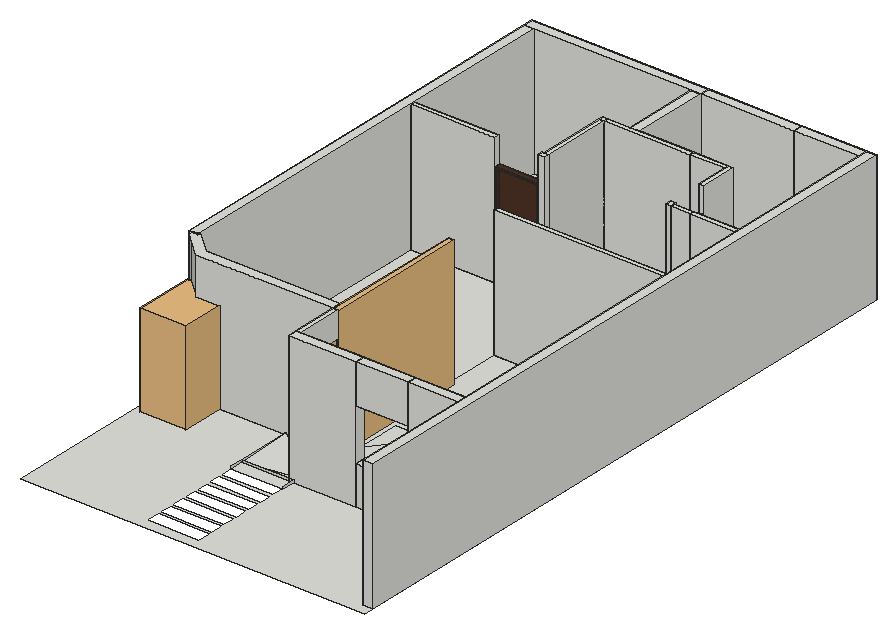
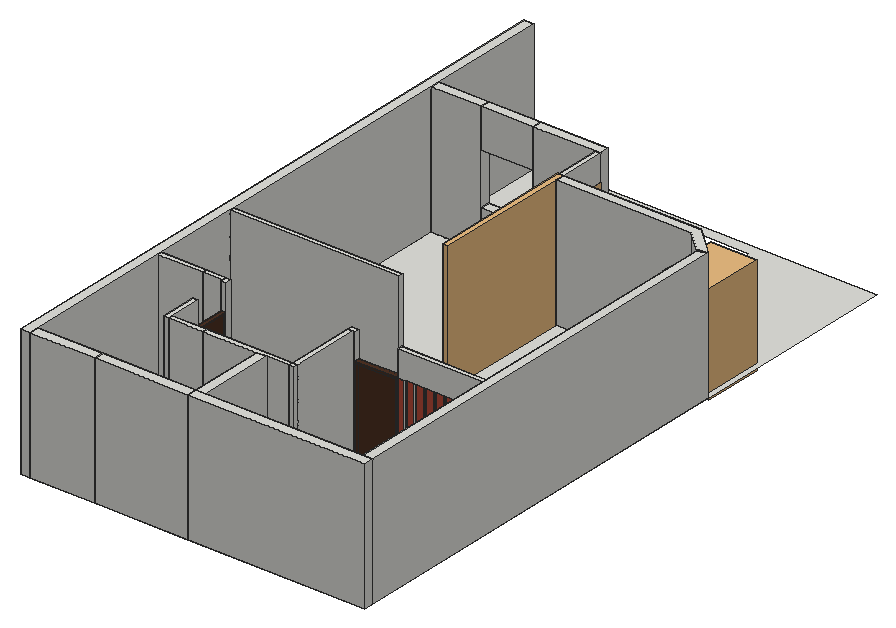
# SketchUp Ruby script. Lengths in inches.
U = 1.inch
M = Sketchup.active_model
def pt(a) = Geom::Point3d.new(a.map { |v| v * U })
def face(e, loops, mat)
  f = e.add_face(loops[0].map { |a| pt(a) })
  loops[1..].each { |l| e.add_face(l.map { |a| pt(a) }).erase! }
  f.material = f.back_material = mat if mat
  f
end
# faces: each face lists its corners as indices into pts; further lists are holes
def faces(e, pts, list, mat = nil) = list.each { |f| face(e, (f[0].is_a?(Array) ? f : [f]).map { |l| l.map { |i| pts[i] } }, mat) }
# xy, xz, yz: faces in a plane at the given z, y or x. An outline is a flat list of corners, or four numbers for a rectangle; further outlines are holes
def ring(l) = l.size == 4 ? [[l[0], l[1]], [l[2], l[1]], [l[2], l[3]], [l[0], l[3]]] : l.each_slice(2).to_a
def flat(e, list, mat, &to3) = list.each { |f| face(e, (f[0].is_a?(Array) ? f : [f]).map { |l| ring(l).map { |u, v| to3.(u, v) } }, mat) }
def xy(e, z, list, mat = nil) = flat(e, list, mat) { |x, y| [x, y, z] }
def xz(e, y, list, mat = nil) = flat(e, list, mat) { |x, z| [x, y, z] }
def yz(e, x, list, mat = nil) = flat(e, list, mat) { |y, z| [x, y, z] }
def lines(e, pts, list) = list.each { |a, b| e.add_line(pt(pts[a]), pt(pts[b])) }
# prism: a flat outline (further loops are holes) pulled along v
def prism(e, loops, v, mat = nil)
  f = face(e, loops, mat); d = Geom::Vector3d.new(v.map { |x| x * U })
  f.pushpull(f.normal.samedirection?(d) ? d.length : -d.length)
end
def box(e, o, s, mat = nil) = prism(e, [[o, [o[0] + s[0], o[1], o[2]], [o[0] + s[0], o[1] + s[1], o[2]], [o[0], o[1] + s[1], o[2]]]], [0, 0, s[2]], mat)
def at(x, y, z, deg = 0) = Geom::Transformation.translation(pt([x, y, z])) * Geom::Transformation.rotation(ORIGIN, Z_AXIS, deg.degrees)
def axes(o, x, y, z) = Geom::Transformation.new([*x, 0, *y, 0, *z, 0, *pt(o).to_a, 1])
def part(name) = M.definitions.add(name)
# library, detail: a bought-in or finely detailed component or shape, given as its bounding box
def library(name, o, s) = part(name).tap { |d| box(d.entities, o, s) }
def detail(e, o, s) = box(e.add_group.entities, o, s)
def put(e, d, t, mat = nil) = e.add_instance(d, t).tap { |i| i.material = mat if mat }
def group(e, t, mat = nil) = e.add_group.tap { |g| g.transformation = t; g.material = mat if mat }.entities
root = M.entities
M.materials.add("Marc_Wrist").color = [188, 79, 61]
M.materials.add("Material1").color = [58, 110, 58]
M.materials.add("Material10").color = [48, 100, 38]
M.materials.add("Material3").color = [68, 110, 58]
M.materials.add("Material4").color = [48, 90, 38]
M.materials.add("Material5").color = [68, 110, 48]
M.materials.add("Material6").color = [48, 90, 48]
M.materials.add("Material8").color = [58, 90, 38]
M.materials.add("Material9").color = [68, 100, 58]
M.materials.add("Polis06_194").color = [79, 50, 36]
M.materials.add("ThomThom - ShoesRubber2").color = [10, 10, 10]
M.materials.add("[Color_E04]").color = [255, 255, 153]
M.materials.add("[Wood Cherry Original]").color = [152, 86, 42]
c1 = part("grass00")
p = [[-0.6875,0.15,0],[-0.56,0.08,5.52],[-0.04,0.03,2.76],[0.48,-0.02,0],[0.35,-0.02,5.52],[-0.1,-0.14,5.52],
  [-0.12,0.65,8.37],[-0.42,0.65,8.37]]
faces(c1.entities,p,[[0,1,2,3],[3,2,4],[1,5,2],[5,4,2],[1,6,5],[4,5,6],[7,6,1]])
c2 = part("Group16\#1")
put(c2.entities,c1,axes([1.44,-0.61,-0.01],[0.05352,0.12609,0],[-0.10704,0.04543,0.07239],[0.06664,-0.02828,0.11628]),"Material6")
put(c2.entities,c1,axes([0.76,-0.15,-0.01],[0.04676,0.24062,0],[-0.23162,0.04501,0.06642],[0.0652,-0.01267,0.23595]),"Material3")
put(c2.entities,c1,axes([0.79,0.01,-0.01],[-0.00606,0.34651,0],[-0.34381,-0.00602,0.0432],[0.04319,0.00076,0.34386]))
put(c2.entities,c1,axes([1,0.23,-0.01],[-0.07192,0.31144,0],[-0.28722,-0.06632,0.1236],[0.12043,0.02781,0.29478]),"Material5")
put(c2.entities,c1,axes([1.66,0.77,-0.01],[-0.13828,0.29651,0],[-0.21551,-0.1005,0.22471],[0.20365,0.09498,0.23779]),"Material10")
put(c2.entities,c1,axes([0.6875,0.52,-0.01],[-0.18126,0.24051,0],[-0.22746,-0.17142,0.09788],[0.07817,0.05891,0.28481]),"Material5")
put(c2.entities,c1,axes([0.68,0.78,-0.01],[-0.215,0.18688,0],[-0.12385,-0.14248,0.21334],[0.13995,0.16101,0.18878]),"Material3")
put(c2.entities,c1,axes([0.56,1,-0.01],[-0.13756,0.07624,0],[-0.06159,-0.11112,0.0927],[0.04494,0.08108,0.12705]),"Material5")
put(c2.entities,c1,axes([0.2,0.64,-0.01],[-0.23729,0.07254,0],[-0.05711,-0.18681,0.153],[0.04473,0.14632,0.19535]),"Material10")
put(c2.entities,c1,axes([0.0625,0.72,-0.01],[-0.28874,0.02525,0],[-0.02179,-0.24916,0.14647],[0.01276,0.14591,0.25012]),"Material3")
put(c2.entities,c1,axes([-0.08,0.62,-0.01],[-0.34089,-0.04187,0],[0.03255,-0.26504,0.216],[-0.02633,0.21439,0.26703]),"Material10")
put(c2.entities,c1,axes([-0.34,0.98,-0.01],[-0.14314,-0.0493,0],[0.04397,-0.12769,0.06843],[-0.02228,0.0647,0.13505]),"Material10")
put(c2.entities,c1,axes([-0.87,1.45,-0.01],[-0.23488,-0.14114,0],[0.13761,-0.22901,0.06087],[-0.03135,0.05217,0.26717]))
put(c2.entities,c1,axes([-0.72,0.77,-0.01],[-0.14208,-0.13251,0],[0.07209,-0.0773,0.16301],[-0.11118,0.11922,0.1057]),"Material10")
put(c2.entities,c1,axes([-0.62,0.43,-0.01],[-0.14845,-0.21203,0],[0.18654,-0.13061,0.12304],[-0.10079,0.07057,0.22772]),"Material3")
put(c2.entities,c1,axes([-0.68,0.29,-0.01],[-0.13639,-0.32136,0],[0.31723,-0.13464,0.05579],[-0.05136,0.0218,0.34462]),"Material4")
put(c2.entities,c1,axes([-0.64,0.125,-0.01],[-0.0458,-0.23569,0],[0.22124,-0.043,0.08276],[-0.08124,0.01579,0.22538]),"Material1")
put(c2.entities,c1,axes([-1.6,-0.03,-0.01],[0.00576,-0.32897,0],[0.27526,0.00482,0.18018],[-0.18015,-0.00315,0.2753]),"Material5")
put(c2.entities,c1,axes([-1.36,-0.31,-0.01],[0.05718,-0.24765,0],[0.18172,0.04196,0.17267],[-0.16825,-0.03885,0.1865]),"Material10")
put(c2.entities,c1,axes([-1.54,-0.72,-0.01],[0.06537,-0.14017,0],[0.13555,0.06321,0.03939],[-0.0357,-0.01665,0.14956]))
put(c2.entities,c1,axes([-1.19,-0.9,-0.01],[0.09597,-0.12735,0],[0.11214,0.08451,0.07557],[-0.06035,-0.04548,0.14042]),"Material9")
put(c2.entities,c1,axes([-0.47,-0.54,-0.01],[0.11588,-0.10072,0],[0.0618,0.0711,0.12124],[-0.07953,-0.0915,0.0942]))
put(c2.entities,c1,axes([-0.47,-0.84,-0.01],[0.11927,-0.0661,0],[0.06603,0.11913,0.00646],[-0.00313,-0.00565,0.13621]),"Material5")
put(c2.entities,c1,axes([-0.38,-1.24,-0.01],[0.28037,-0.08571,0],[0.0618,0.20215,0.20315],[-0.05939,-0.19428,0.21139]),"Material9")
put(c2.entities,c1,axes([-0.06,-0.66,-0.01],[0.22719,-0.01987,0],[0.01247,0.14255,0.17758],[-0.01547,-0.17691,0.1431]),"Material8")
put(c2.entities,c1,axes([0.11,-0.89,-0.01],[0.14882,0.01828,0],[-0.01058,0.08611,0.12229],[0.01491,-0.12138,0.08676]),"Material6")
put(c2.entities,c1,axes([0.25,-0.72,-0.01],[0.20481,0.07053,0],[-0.06206,0.18022,0.10291],[0.03351,-0.0973,0.1906]),"Material6")
put(c2.entities,c1,axes([0.85,-1.42,-0.01],[0.16481,0.09904,0],[-0.09472,0.15762,0.05616],[0.02893,-0.04814,0.18389]),"Material5")
put(c2.entities,c1,axes([1.01,-1.09,-0.01],[0.21858,0.20385,0],[-0.17495,0.1876,0.15339],[0.10462,-0.11218,0.25652]),"Material10")
put(c2.entities,c1,axes([1.01,-0.71,-0.01],[0.08733,0.12473,0],[-0.06445,0.04512,0.13037],[0.1068,-0.07477,0.07867]),"Material6")
c3 = part("Group15\#1")
put(c3.entities,c2,at(0,0,0))
c4 = part("3darcstudiotree_grass00\#1")
put(c4.entities,c3,at(0,0,0))
c5 = library("DD LT 2",[0,0,0],[47.24,4.7,78.74])
c6 = library("Group\#96",[-3.28,-8.3,0],[42.48,54.86,91.86])
c7 = library("Group\#9",[0,0,0],[5.16,133,120])
c8 = part("Group\#23")
box(c8.entities,[0,0,0],[12.05,39.48,6])
c9 = part("Flush door")
xy(c9.entities,0,[[0,0,4.72,1.18],[0,34.25,4.72,35.43]],"Polis06_194")
xy(c9.entities,85.26,[[0,1.18,4.72,34.25]],"Polis06_194")
xy(c9.entities,86.61,[[0,0,4.72,35.43]],"Polis06_194")
xz(c9.entities,0,[[0,0,4.72,86.61]],"Polis06_194")
xz(c9.entities,1.18,[[0,0,2.36,85.26],[2.36,0,4.72,85.26]],"Polis06_194")
xz(c9.entities,34.25,[[0,0,4.72,85.26]],"Polis06_194")
xz(c9.entities,35.43,[[0,0,4.72,86.61]],"Polis06_194")
yz(c9.entities,0,[[0,0,1.18,86.61],[34.25,0,35.43,86.61],[1.18,85.26,34.25,86.61]],"Polis06_194")
yz(c9.entities,2.36,[[1.18,0,34.25,0,34.25,85.21,1.18,85.26]],"Polis06_194")
yz(c9.entities,4.72,[[0,0,1.18,86.61],[34.25,0,35.43,86.61],[1.18,85.26,34.25,86.61]],"Polis06_194")
xy(root,0,[[[28.97,48,346.97,638.5],[138.47,142.5,138.47,166.5,191.85,175.5,181.97,175.5,181.97,403.5,337.97,403.5,337.97,175.5,223.49,175.5,181.66,166.5,186.47,166.5,186.47,142.5],[138.47,57,186.47,70.5],[138.47,72.5,186.47,84.5],[138.47,86.5,186.47,98.5],[138.47,100.5,186.47,112.5],[138.47,114.5,186.47,126.5],[138.47,128.5,186.47,140.5]],[138.47,154.5,186.47,166.5],[138.47,166.5,191.85,175.5,223.49,175.5,181.66,166.5],[181.97,175.5,181.97,403.5,337.97,403.5,337.97,175.5,223.49,175.5,223.49,277.625,191.85,277.625,191.85,175.5],[191.85,175.5,223.49,277.625]])
xz(root,166.5,[[138.47,0,181.66,2],[181.66,0,186.47,2]])
yz(root,138.47,[[154.5,0,166.5,2],[166.5,0,166.5,2,218,2]])
yz(root,186.47,[[154.5,0,166.5,2]])
p = [[191.85,175.5,0],[138.47,166.5,0],[138.47,218,2],[181.66,166.5,0],[223.49,175.5,0],[181.66,166.5,2],
  [223.49,277.625,0],[181.66,218,2]]
faces(root,p,[[0,1,2],[3,4,5],[5,4,6,7]])
put(root,c4,axes([269.28,156.1,0.25],[-0.22387,-0.80552,0],[1.0592,-0.20279,-0.03351],[0.04802,-0.00919,1.59864]))
put(root,c4,axes([290.93,156.19,0.25],[0.49112,-0.73053,0],[0.87176,0.40374,-0.05199],[0.06457,0.02991,1.41973]))
put(root,c4,axes([284.67,156.17,0.25],[-0.12943,-0.86251,0],[1.22125,-0.12625,-0.06365],[0.09727,-0.01005,1.89522]))
put(root,c4,axes([279.83,156.25,0.25],[1.20229,-0.17424,0],[0.22233,1.05686,-0.04063],[0.0079,0.03755,1.46079]))
put(root,c4,axes([272.69,156.16,0.25],[1.1073,0.16654,0],[-0.19879,0.91056,-0.0513],[-0.01271,0.0582,1.54883]))
put(root,c4,axes([320.76,156.41,0.25],[1.01668,-0.29704,0],[0.42792,1.009,-0.03514],[0.01412,0.0333,1.55988]))
put(root,c4,axes([305.95,156.15,0.25],[0.65905,0.58136,0],[-0.67112,0.52412,-0.04643],[-0.06422,0.05015,1.7498]))
put(root,c4,axes([326.7,156.44,0.25],[0.29173,-0.98541,0],[1.06443,0.21709,-0.05295],[0.09268,0.0189,1.97565]))
put(root,c4,axes([311.92,156.23,0.25],[-1.12473,-0.36385,0],[0.38499,-0.81984,-0.03755],[0.02004,-0.04268,1.55797]))
put(root,c4,axes([316.25,156.44,0.25],[0.97955,0.1289,0],[-0.18056,0.94523,-0.02805],[-0.0076,0.03978,1.99488]))
put(root,c4,axes([328.6,156.33,0.25],[-1.09984,-0.09953,0],[0.11105,-0.84533,-0.05296],[0.00908,-0.06913,1.62079]))
put(root,c4,axes([313.35,156.93,0.25],[0.25876,-0.96087,0],[1.1152,0.20689,-0.0396],[0.05023,0.00932,1.48525]))
put(root,c4,axes([327.01,156.98,0.25],[1.05284,-0.01508,0],[0.02011,0.96713,-0.0287],[0.00084,0.04054,1.98369]))
put(root,c4,axes([293.45,157.05,0.25],[0.29225,-0.8464,0],[1.03075,0.24519,-0.03571],[0.06278,0.01493,1.9611]))
put(root,c4,axes([320.57,157.11,0.25],[0.53762,-0.86689,0],[1.12439,0.48038,-0.06088],[0.07123,0.03043,1.6642]))
put(root,c4,axes([324.09,157.08,0.25],[0.96968,-0.15073,0],[0.21991,0.97464,-0.05648],[0.01218,0.05398,1.39957]))
put(root,c4,axes([315.95,157.2,0.25],[0.27192,-0.91374,0],[1.08554,0.22255,-0.04714],[0.05499,0.01127,1.34372]))
put(root,c4,axes([275.21,157.2,0.25],[1.08689,0.01633,0],[-0.02208,1.01203,-0.04973],[-0.0014,0.0643,1.89995]))
put(root,c4,axes([276.67,157.19,0.25],[-0.8707,-0.72263,0],[0.80748,-0.67025,-0.05204],[0.0571,-0.0474,1.77215]))
put(root,c4,axes([312.01,157.28,0.25],[-0.12355,-0.76842,0],[1.15696,-0.12815,-0.03174],[0.04792,-0.00531,1.77768]))
put(root,c4,axes([278.2,157.26,0.25],[1.00504,0.56503,0],[-0.7161,0.87749,-0.02464],[-0.02146,0.02629,1.98292]))
put(root,c4,axes([287.13,157.4,0.25],[0.45874,-0.78763,0],[0.96539,0.38735,-0.03335],[0.04481,0.01798,1.60043]))
put(root,c4,axes([308.2,157.3,0.25],[-0.78015,-0.39287,0],[0.593,-0.81123,-0.04577],[0.04071,-0.05569,1.96036]))
put(root,c4,axes([295.24,157.52,0.25],[0.54893,-0.66037,0],[0.82145,0.4704,-0.0362],[0.05761,0.03299,1.92943]))
put(root,c4,axes([329.52,157.2,0.25],[-0.91686,0.36615,0],[-0.49157,-0.84799,-0.05656],[-0.0334,-0.05762,1.54444]))
put(root,c4,axes([269.0625,157.21,0.25],[-0.75365,0.4777,0],[-0.72678,-0.7899,-0.0597],[-0.0585,-0.06358,1.93343]))
put(root,c4,axes([272.05,157.36,0.25],[0.83304,0.68517,0],[-0.9025,0.75592,-0.05903],[-0.05961,0.04993,1.83956]))
put(root,c4,axes([310.37,157.58,0.25],[0.65458,-0.59511,0],[0.82814,0.62752,-0.05494],[0.06642,0.05033,1.83588]))
put(root,c4,axes([328.48,157.23,0.25],[-0.62961,0.7944,0],[-1.037,-0.5662,-0.04701],[-0.0514,-0.02807,1.62457]))
put(root,c4,axes([299.27,157.36,0.25],[0.08246,0.90458,0],[-1.02646,0.06446,-0.04286],[-0.05913,0.00371,1.42447]))
put(root,c4,axes([273.44,157.8,0.25],[0.59852,-0.79757,0],[0.94427,0.48816,-0.04551],[0.05811,0.03004,1.67334]))
put(root,c4,axes([267.45,157.62,0.25],[-0.98051,-0.24115,0],[0.29451,-0.82493,-0.05017],[0.02121,-0.0594,1.54202]))
put(root,c4,axes([284.89,157.5625,0.25],[-0.95921,0.3162,0],[-0.37509,-0.78387,-0.04199],[-0.0257,-0.05371,1.68502]))
put(root,c4,axes([288.875,157.6,0.25],[0.39945,0.97742,0],[-1.1292,0.31792,-0.04327],[-0.06048,0.01703,1.7601]))
put(root,c4,axes([296.08,157.67,0.25],[-0.06561,0.8087,0],[-1.0841,-0.06059,-0.04305],[-0.07067,-0.00395,1.78778]))
put(root,c4,axes([303.16,157.68,0.25],[-0.01182,0.91075,0],[-1.29491,-0.01157,-0.05791],[-0.07195,-0.00064,1.60897]))
put(root,c4,axes([297.99,157.83,0.25],[-0.96542,-0.01081,0],[0.01408,-0.86615,-0.03579],[0.00074,-0.04576,1.60809]))
put(root,c4,axes([318.17,157.76,0.25],[-0.53234,0.80865,0],[-1.08104,-0.49026,-0.04785],[-0.06058,-0.02747,1.77706]))
put(root,c4,axes([310.57,158.37,0.25],[-0.0774,-0.99652,0],[1.26825,-0.06786,-0.03565],[0.04285,-0.00229,1.53082]))
put(root,c4,axes([285.65,158.4,0.25],[1.05948,-0.19855,0],[0.21799,0.80133,-0.03599],[0.01059,0.03891,1.32194]))
put(root,c4,axes([301.56,158.32,0.25],[-1.00494,-0.55943,0],[0.51605,-0.63861,-0.03319],[0.03265,-0.0404,1.63594]))
put(root,c4,axes([299.49,158.55,0.25],[0.95997,-0.61983,0],[0.77038,0.82195,-0.05588],[0.04568,0.04874,1.67045]))
put(root,c4,axes([314.6875,158.35,0.25],[0.93611,0.65761,0],[-0.73196,0.71779,-0.04954],[-0.05043,0.04945,1.78537]))
put(root,c4,axes([317.24,158.63,0.25],[0.51232,-0.95574,0],[0.91823,0.33908,-0.03607],[0.0464,0.01713,1.41495]))
put(root,c4,axes([332.48,158.62,0.25],[0.82557,-0.8273,0],[0.72903,0.50118,-0.04892],[0.06335,0.04355,1.59182]))
put(root,c4,axes([330.11,158.25,0.25],[-0.88156,0.44778,0],[-0.58548,-0.79407,-0.04749],[-0.02897,-0.03928,1.3106]))
put(root,c4,axes([291.8125,158.49,0.25],[-0.81808,-0.31568,0],[0.4026,-0.71875,-0.04575],[0.03238,-0.0578,1.60296]))
put(root,c4,axes([312.04,158.7,0.25],[-0.67997,-0.91004,0],[0.92657,-0.47694,-0.05324],[0.07665,-0.03946,1.84703]))
put(root,c4,axes([273.88,158.82,0.25],[0.07392,-0.80055,0],[1.1197,0.07122,-0.05496],[0.09372,0.00596,1.9204]))
put(root,c4,axes([289.9375,158.63,0.25],[-0.90907,-0.51539,0],[0.73237,-0.8899,-0.03279],[0.02416,-0.02935,1.69581]))
put(root,c4,axes([269.81,158.83,0.25],[0.94047,0.12054,0],[-0.15763,0.84725,-0.03647],[-0.00846,0.04546,1.56991]))
put(root,c4,axes([305.34,158.74,0.25],[0.66709,0.83909,0],[-0.77262,0.42315,-0.04277],[-0.06119,0.03351,1.58679]))
put(root,c4,axes([289.11,158.93,0.25],[-0.58234,-0.63321,0],[0.77276,-0.48958,-0.04177],[0.04676,-0.02962,1.36919]))
put(root,c4,axes([277.8,158.91,0.25],[-0.89035,-0.49536,0],[0.64432,-0.7978,-0.05337],[0.04071,-0.05041,1.58535]))
put(root,c4,axes([312.77,158.81,0.25],[-0.70141,0.49254,0],[-0.79786,-0.78274,-0.04396],[-0.0419,-0.04111,1.82298]))
put(root,c4,axes([304.35,158.92,0.25],[-0.0259,1.03945,0],[-1.26909,-0.02178,-0.04199],[-0.0557,-0.00096,1.68448]))
put(root,c4,axes([281.79,159.4375,0.25],[-0.72108,-0.89684,0],[0.82715,-0.45815,-0.04802],[0.06823,-0.03779,1.69851]))
put(root,c4,axes([304.04,159.55,0.25],[1.13425,-0.32694,0],[0.4029,0.96294,-0.03586],[0.01728,0.04129,1.80381]))
put(root,c4,axes([325.71,159.59,0.25],[0.66638,-0.84913,0],[1.08193,0.58493,-0.04483],[0.04836,0.02615,1.66248]))
put(root,c4,axes([276.74,159.49,0.25],[-0.19052,-0.74327,0],[1.05272,-0.1859,-0.04713],[0.06782,-0.01198,1.58351]))
put(root,c4,axes([280.39,159.55,0.25],[1.17952,-0.13892,0],[0.16881,0.98743,-0.05794],[0.01236,0.07231,1.82474]))
put(root,c4,axes([305.98,159.625,0.25],[0.60406,-0.56523,0],[0.91749,0.67548,-0.037],[0.0345,0.0254,1.52862]))
put(root,c4,axes([275.68,159.81,0.25],[0.92463,-0.01843,0],[0.02797,0.9665,-0.04057],[0.00112,0.03868,1.33829]))
put(root,c4,axes([331.92,159.61,0.25],[0.21335,1.005,0],[-1.17496,0.17183,-0.04576],[-0.06227,0.00911,1.64855]))
put(root,c4,axes([302.26,159.84,0.25],[-0.8364,-0.44999,0],[0.56519,-0.72371,-0.04254],[0.03985,-0.05103,1.78955]))
put(root,c4,axes([271.84,160.04,0.25],[0.64014,-0.81698,0],[0.77801,0.41995,-0.04791],[0.07635,0.04121,1.76421]))
put(root,c4,axes([323.8125,159.72,0.25],[-0.26521,0.85563,0],[-1.24374,-0.26558,-0.03008],[-0.04009,-0.00856,1.76703]))
put(root,c4,axes([295.34,159.9,0.25],[0.66676,0.61243,0],[-0.78466,0.58851,-0.0306],[-0.04003,0.03002,1.86488]))
put(root,c4,axes([285.49,159.83,0.25],[0.10899,0.86828,0],[-1.08137,0.09351,-0.02993],[-0.04423,0.00383,1.61572]))
put(root,c4,axes([308.8,159.875,0.25],[-1.23168,0.08712,0],[-0.08586,-0.83621,-0.04489],[-0.00703,-0.06843,1.86365]))
put(root,c4,axes([271.13,159.95,0.25],[-0.89059,-0.35165,0],[0.52311,-0.91269,-0.03826],[0.02469,-0.04308,1.82966]))
put(root,c4,axes([320.75,159.9,0.25],[-0.93761,-0.01602,0],[0.02628,-1.05964,-0.05231],[0.00161,-0.06486,1.90792]))
put(root,c4,axes([268.29,159.93,0.25],[-0.57666,0.88438,0],[-1.05888,-0.47564,-0.04902],[-0.06326,-0.02842,1.76654]))
put(root,c4,axes([329.43,160.09,0.25],[0.76693,0.86238,0],[-0.77032,0.47194,-0.03251],[-0.04482,0.02746,1.64081]))
put(root,c4,axes([293.15,160.17,0.25],[-0.80928,-0.52621,0],[0.66742,-0.70711,-0.04081],[0.03405,-0.03607,1.46417]))
put(root,c4,axes([301.26,160.04,0.25],[-0.75344,0.4177,0],[-0.57005,-0.70837,-0.04884],[-0.03669,-0.04559,1.38796]))
put(root,c4,axes([268.94,160.22,0.25],[-0.46931,0.75093,0],[-1.01019,-0.43493,-0.04385],[-0.04839,-0.02083,1.41492]))
put(root,c4,axes([286.92,160.28,0.25],[-1.11875,0.33955,0],[-0.31517,-0.71537,-0.04181],[-0.02149,-0.04878,1.37365]))
put(root,c4,axes([290.07,160.33,0.25],[0.17128,1.04977,0],[-1.22313,0.13749,-0.03426],[-0.04872,0.00548,1.77113]))
put(root,c4,axes([326.93,160.34,0.25],[-0.64812,0.54043,0],[-0.6442,-0.53223,-0.04592],[-0.0512,-0.0423,1.42994]))
put(root,c4,axes([271.09,160.76,0.25],[0.65433,-0.72199,0],[0.97287,0.6074,-0.05537],[0.05486,0.03425,1.50911]))
put(root,c4,axes([289.0625,160.7,0.25],[1.0835,-0.06808,0],[0.07893,0.86532,-0.04662],[0.00566,0.06203,1.68074]))
put(root,c4,axes([315.71,160.71,0.25],[0.96359,0.58622,0],[-0.70206,0.795,-0.04132],[-0.03872,0.04384,1.88254]))
put(root,c4,axes([307.38,161.03,0.25],[1.16574,-0.27548,0],[0.29636,0.86396,-0.0361],[0.0137,0.03993,1.4995]))
put(root,c4,axes([279.82,160.7,0.25],[-0.546,0.83334,0],[-0.90556,-0.40874,-0.03157],[-0.04848,-0.02188,1.80167]))
put(root,c4,axes([285.73,160.79,0.25],[0.04965,0.93178,0],[-1.05803,0.03884,-0.03464],[-0.05115,0.00188,1.56527]))
put(root,c4,axes([278.58,161.1,0.25],[0.95118,0.11266,0],[-0.16799,0.97704,-0.03434],[-0.00697,0.04053,1.70799]))
put(root,c4,axes([300.8,161.07,0.25],[0.98116,0.22946,0],[-0.33667,0.99174,-0.04858],[-0.0167,0.0492,1.57379]))
put(root,c4,axes([290.61,160.74,0.25],[-0.59566,0.95582,0],[-1.08814,-0.46716,-0.04288],[-0.05248,-0.02253,1.68813]))
put(root,c4,axes([312.24,160.79,0.25],[-0.9635,0.59263,0],[-0.67846,-0.75989,-0.03727],[-0.03661,-0.04101,1.88005]))
put(root,c4,axes([272.3,160.89,0.25],[-0.47452,0.74232,0],[-1.01345,-0.4463,-0.05129],[-0.05297,-0.02332,1.34106]))
put(root,c4,axes([296.42,161.3,0.25],[0.70875,-0.73014,0],[0.76813,0.51366,-0.02709],[0.03876,0.02592,1.8123]))
put(root,c4,axes([318.03,161.32,0.25],[0.94895,-0.19935,0],[0.28745,0.94267,-0.03471],[0.01406,0.04611,1.93398]))
put(root,c4,axes([293.3,161.28,0.25],[-0.11715,-0.7811,0],[1.21875,-0.12592,-0.05859],[0.08691,-0.00898,1.83593]))
put(root,c4,axes([332.66,161.01,0.25],[-0.50258,0.73326,0],[-0.8921,-0.42123,-0.04597],[-0.05154,-0.02434,1.32398]))
put(root,c4,axes([324.8,161.36,0.25],[1.03956,-0.1215,0],[0.14171,0.83528,-0.04526],[0.01113,0.06561,1.7925]))
put(root,c4,axes([313.47,161.33,0.25],[-0.74357,-0.80548,0],[0.96193,-0.61175,-0.04805],[0.05089,-0.03236,1.61679]))
put(root,c4,axes([323.46,161.14,0.25],[-0.31136,0.90043,0],[-0.89194,-0.21247,-0.04255],[-0.07759,-0.01848,1.76068]))
put(root,c4,axes([329.57,161.23,0.25],[-0.90955,0.3659,0],[-0.39974,-0.68453,-0.04774],[-0.03777,-0.06468,1.66266]))
put(root,c4,axes([267.78,161.37,0.25],[-0.7325,-0.56683,0],[0.76421,-0.68034,-0.04642],[0.04267,-0.03799,1.51042]))
put(root,c4,axes([284.07,161.52,0.25],[-0.24653,-1.01305,0],[1.11137,-0.18632,-0.03802],[0.05876,-0.00985,1.78771]))
put(root,c4,axes([315.13,161.3125,0.25],[-1.1689,0.03052,0],[-0.03131,-0.82623,-0.03177],[-0.00199,-0.05252,1.98473]))
put(root,c4,axes([297.89,161.57,0.25],[-0.83168,0.53002,0],[-0.68594,-0.7415,-0.05552],[-0.04904,-0.05301,1.63365]))
put(root,c4,axes([298.15,162,0.25],[0.59558,-0.79038,0],[0.80082,0.41572,-0.0272],[0.04442,0.02306,1.81972]))
put(root,c4,axes([319.22,161.99,0.25],[0.37663,-0.6948,0],[1.07253,0.40052,-0.04402],[0.06207,0.02318,1.81837]))
put(root,c4,axes([325.3,161.9375,0.25],[0.98525,0.26801,0],[-0.36328,0.91998,-0.04711],[-0.01959,0.04961,1.55738]))
put(root,c4,axes([304.3,162.0625,0.25],[-0.43691,-0.6584,0],[1.12851,-0.51591,-0.06742],[0.07245,-0.03312,1.58058]))
put(root,c4,axes([332.61,162.29,0.25],[0.99168,-0.39467,0],[0.41553,0.71928,-0.03326],[0.02459,0.04256,1.64345]))
put(root,c4,axes([273.96,162.36,0.25],[-0.66171,-0.6274,0],[0.92907,-0.67503,-0.03006],[0.03174,-0.02306,1.73276]))
put(root,c4,axes([308.32,162.23,0.25],[0.06923,0.88101,0],[-0.99259,0.05373,-0.03468],[-0.05993,0.00324,1.72254]))
g1 = group(root,at(291.92,166.5,0))
box(g1,[0,0,0],[46.05,9,120])
g2 = group(root,at(243.92,166.5,0))
box(g2,[0,0,0],[48,9,36])
box(g2,[0,0,84],[48,9,36])
p = [[48,9,36],[48,9,84],[0,9,36],[0,9,84]]
lines(g2,p,[[0,1],[2,3]])
g3 = group(root,at(186.47,166.5,0))
box(g3,[-4.81,0,0],[62.26,9,120])
put(root,c5,axes([180.9,217.74,0],[0.00003,-0.89406,0],[0.6897,0.00003,0],[0.00001,0,1.21]))
g4 = group(root,at(181.66,175.5,0))
prism(g4,[[[4.5,0,120],[4.5,0,96],[4.5,42.24,96],[4.5,42.24,0],[4.5,42.5,0],[4.5,42.5,120]]],[-4.5,0,0])
put(root,c6,at(37.66,187.6875,-6.78))
g5 = group(root,at(28.97,218,0))
prism(g5,[[[9,26.34,0],[28.05,9,0],[153,9,0],[153,0,0],[26.31,0,0],[9,15.76,0],[0,23.95,0],[9,23.95,0]]],[0,0,120])
g6 = group(root,at(28.97,241.95,0))
prism(g6,[[[0,0,0],[9,2.39,0],[9,0,0]]],[0,0,120])
put(root,c7,at(181.97,218,0))
g7 = group(root,at(337.97,57,0))
prism(g7,[[[0,572.5,0],[0,581.5,0],[9,581.5,0],[9,0,0],[0,0,0],[0,109.5,0],[0,118.5,0],[0,346.5,0],[0,351,0]]],[0,0,120])
g8 = group(root,at(181.97,403.5,0))
box(g8,[0,0,0],[156,4.5,120])
g9 = group(root,at(28.97,241.95,0))
prism(g9,[[[0,0,0],[0,387.55,0],[9,387.55,0],[9,249.55,0],[9,245.05,0],[9,2.39,0]]],[0,0,120])
put(root,c8,at(184.6,447.38,0))
g10 = group(root,at(277.97,487,0))
box(g10,[0,0,0],[17.9,4.5,120])
g11 = group(root,at(155.85,487,0))
prism(g11,[[[6.62,4.5,0],[6.62,0,0],[0,0,0],[0,4.5,0],[2.12,4.5,0]]],[0,0,120])
g12 = group(root,at(295.87,487,0))
box(g12,[0,0,0],[42.1,4.5,120])
put(root,c9,axes([116.3,491.93,0],[0,-1.043,0],[1.11623,0,0],[0,0,1.10836]))
g13 = group(root,at(273.47,487,0))
box(g13,[0,0,0],[4.5,6.55,120])
g14 = group(root,at(37.97,487,0))
xy(g14,0,[[0,0,0,4.83,5.88,4.83,5.88,4.5,71.91,4.5,71.91,4.83,77.88,4.83,77.88,0]])
xy(g14,13.4,[[5.88,4.5,71.91,10.5]])
xy(g14,21.31,[[5.88,4.5,7.88,4.5,7.88,4.83,15.03,4.83,15.03,4.5,17.03,4.5,17.03,4.83,24.17,4.83,24.17,4.5,26.17,4.5,26.17,4.83,33.32,4.83,33.32,4.5,35.32,4.5,35.32,4.83,42.47,4.83,42.47,4.5,44.47,4.5,44.47,4.83,51.61,4.83,51.61,4.5,53.61,4.5,53.61,4.83,60.76,4.83,60.76,4.5,62.76,4.5,62.76,4.83,69.91,4.83,69.91,4.5,71.91,4.5,71.91,10.5,5.88,10.5]],"[Wood Cherry Original]")
xy(g14,96,[[0,4.5,5.88,4.83],[7.88,4.5,15.03,4.83],[17.03,4.5,24.17,4.83],[26.17,4.5,33.32,4.83],[35.32,4.5,42.47,4.83],
  [44.47,4.5,51.61,4.83],[53.61,4.5,60.76,4.83],[62.76,4.5,69.91,4.83],[71.91,4.5,77.88,4.83]])
xy(g14,120,[[0,0,77.88,4.5]])
xz(g14,0,[[0,0,77.88,120]])
xz(g14,4.5,[[0,96,77.88,120]])
xz(g14,4.5,[[7.88,0,15.03,13.4],[17.03,0,24.17,13.4],[26.17,0,33.32,13.4],[35.32,0,42.47,13.4],[44.47,0,51.61,13.4],
  [53.61,0,60.76,13.4],[62.76,0,69.91,13.4]],"Marc_Wrist")
xz(g14,4.5,[[5.88,0,7.88,13.4],[15.03,0,17.03,13.4],[24.17,0,26.17,13.4],[33.32,0,35.32,13.4],[42.47,0,44.47,13.4],
  [51.61,0,53.61,13.4],[60.76,0,62.76,13.4],[69.91,0,71.91,13.4],[5.88,21.31,7.88,96],[15.03,21.31,17.03,96],
  [24.17,21.31,26.17,96],[33.32,21.31,35.32,96],[42.47,21.31,44.47,96],[51.61,21.31,53.61,96],[60.76,21.31,62.76,96],
  [69.91,21.31,71.91,96]],"[Color_E04]")
xz(g14,4.83,[[0,0,5.88,96],[71.91,0,77.88,96],[7.88,21.31,15.03,96],[17.03,21.31,24.17,96],[26.17,21.31,33.32,96],
  [35.32,21.31,42.47,96],[44.47,21.31,51.61,96],[53.61,21.31,60.76,96],[62.76,21.31,69.91,96]],"Marc_Wrist")
xz(g14,10.5,[[[5.88,13.4,71.91,21.31],[6.54,14.0625,71.25,20.65]],[40.17,14.0625,40.7,20.65]],"ThomThom - ShoesRubber2")
xz(g14,10.5,[[6.54,14.0625,40.17,20.65],[40.7,14.0625,71.25,20.65]],"[Wood Cherry Original]")
yz(g14,0,[[0,0,0,120,4.5,120,4.5,96,4.83,96,4.83,0]])
yz(g14,5.88,[[4.5,0,4.83,13.4],[4.83,13.4,10.5,21.31],[4.5,21.31,4.83,96]])
yz(g14,7.88,[[4.5,21.31,4.83,96]])
yz(g14,15.03,[[4.5,21.31,4.83,96]])
yz(g14,17.03,[[4.5,21.31,4.83,96]])
yz(g14,24.17,[[4.5,21.31,4.83,96]])
yz(g14,26.17,[[4.5,21.31,4.83,96]])
yz(g14,33.32,[[4.5,21.31,4.83,96]])
yz(g14,35.32,[[4.5,21.31,4.83,96]])
yz(g14,42.47,[[4.5,21.31,4.83,96]])
yz(g14,44.47,[[4.5,21.31,4.83,96]])
yz(g14,51.61,[[4.5,21.31,4.83,96]])
yz(g14,53.61,[[4.5,21.31,4.83,96]])
yz(g14,60.76,[[4.5,21.31,4.83,96]])
yz(g14,62.76,[[4.5,21.31,4.83,96]])
yz(g14,69.91,[[4.5,21.31,4.83,96]])
yz(g14,71.91,[[4.5,0,4.83,13.4],[4.83,13.4,10.5,21.31],[4.5,21.31,4.83,96]])
yz(g14,77.88,[[0,0,4.83,0,4.83,96,4.5,96,4.5,120,0,120]])
p = [[0,4.5,96],[-0.25,4.5,96]]
lines(g14,p,[[0,1]])
put(root,c9,axes([273.47,493.55,0],[0.7,0,0],[0,0.9075,0],[0,0,1.10836]))
g15 = group(root,at(157.97,491.5,0))
box(g15,[0,0,0],[4.5,63.5,120])
g16 = group(root,at(273.47,525.71,0))
prism(g16,[[[0,29.29,0],[0,33.79,0],[4.5,33.79,0],[4.5,0,0],[0,0,0]]],[0,0,120])
g17 = group(root,at(241.47,555,0))
box(g17,[0,0,0],[32,4.5,120])
g18 = group(root,at(162.47,555,0))
prism(g18,[[[0,0,0],[0,4.5,0],[20.5,4.5,0],[29.5,4.5,0],[79,4.5,0],[79,0,0]]],[0,0,120])
g19 = group(root,at(157.97,555,0))
box(g19,[0,0,0],[4.5,4.5,120])
g20 = group(root,at(182.97,559.5,0))
box(g20,[0,0,0],[9,70,120])
g21 = group(root,at(28.97,629.5,0))
prism(g21,[[[0,0,0],[0,9,0],[163,9,0],[163,0,0],[154,0,0],[9,0,0]]],[0,0,120])
g22 = group(root,at(191.97,629.5,0))
box(g22,[0,0,0],[85.94,9,120])
g23 = group(root,at(277.92,629.5,0))
box(g23,[0,0,0],[60.06,9,120])
